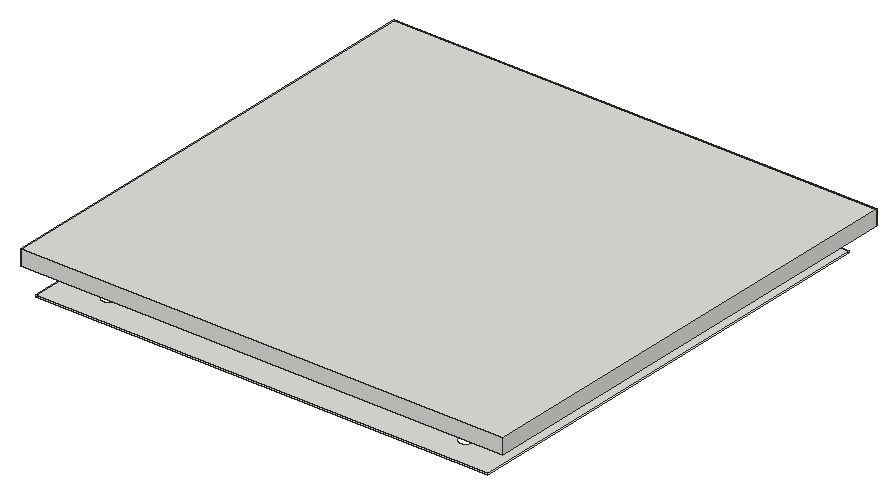
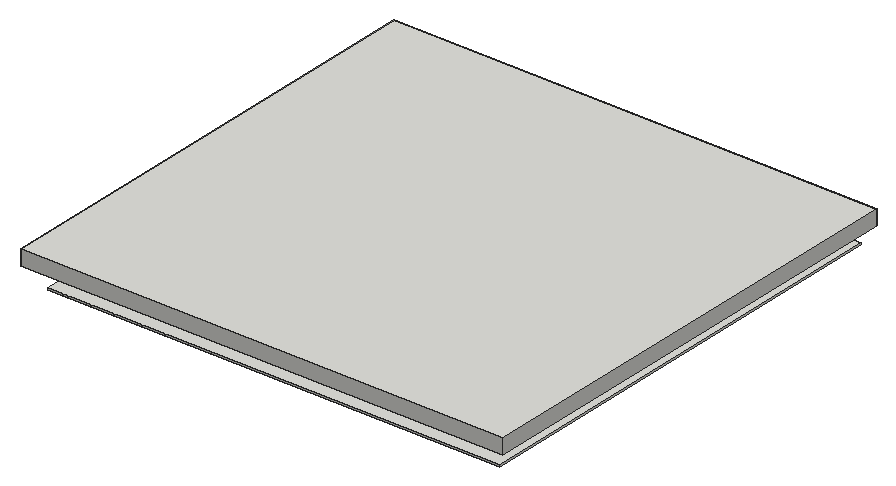
# SketchUp Ruby script. Lengths in inches.
U = 1.inch
M = Sketchup.active_model
def pt(a) = Geom::Point3d.new(a.map { |v| v * U })
def face(e, loops, mat)
  f = e.add_face(loops[0].map { |a| pt(a) })
  loops[1..].each { |l| e.add_face(l.map { |a| pt(a) }).erase! }
  f.material = f.back_material = mat if mat
  f
end
# faces: each face lists its corners as indices into pts; further lists are holes
def faces(e, pts, list, mat = nil) = list.each { |f| face(e, (f[0].is_a?(Array) ? f : [f]).map { |l| l.map { |i| pts[i] } }, mat) }
# xy, xz, yz: faces in a plane at the given z, y or x. An outline is a flat list of corners, or four numbers for a rectangle; further outlines are holes
def ring(l) = l.size == 4 ? [[l[0], l[1]], [l[2], l[1]], [l[2], l[3]], [l[0], l[3]]] : l.each_slice(2).to_a
def flat(e, list, mat, &to3) = list.each { |f| face(e, (f[0].is_a?(Array) ? f : [f]).map { |l| ring(l).map { |u, v| to3.(u, v) } }, mat) }
def xy(e, z, list, mat = nil) = flat(e, list, mat) { |x, y| [x, y, z] }
def xz(e, y, list, mat = nil) = flat(e, list, mat) { |x, z| [x, y, z] }
def yz(e, x, list, mat = nil) = flat(e, list, mat) { |y, z| [x, y, z] }
def lines(e, pts, list) = list.each { |a, b| e.add_line(pt(pts[a]), pt(pts[b])) }
# prism: a flat outline (further loops are holes) pulled along v
def prism(e, loops, v, mat = nil)
  f = face(e, loops, mat); d = Geom::Vector3d.new(v.map { |x| x * U })
  f.pushpull(f.normal.samedirection?(d) ? d.length : -d.length)
end
def box(e, o, s, mat = nil) = prism(e, [[o, [o[0] + s[0], o[1], o[2]], [o[0] + s[0], o[1] + s[1], o[2]], [o[0], o[1] + s[1], o[2]]]], [0, 0, s[2]], mat)
def at(x, y, z, deg = 0) = Geom::Transformation.translation(pt([x, y, z])) * Geom::Transformation.rotation(ORIGIN, Z_AXIS, deg.degrees)
def axes(o, x, y, z) = Geom::Transformation.new([*x, 0, *y, 0, *z, 0, *pt(o).to_a, 1])
def part(name) = M.definitions.add(name)
# library, detail: a bought-in or finely detailed component or shape, given as its bounding box
def library(name, o, s) = part(name).tap { |d| box(d.entities, o, s) }
def detail(e, o, s) = box(e.add_group.entities, o, s)
def put(e, d, t, mat = nil) = e.add_instance(d, t).tap { |i| i.material = mat if mat }
def group(e, t, mat = nil) = e.add_group.tap { |g| g.transformation = t; g.material = mat if mat }.entities
root = M.entities
xy(root,114,[[[4,0,124,120],[28,20,100,96],[112.03,72.63,112.26,72.64,112.48,72.68,112.71,72.74,112.92,72.83,113.125,72.9375,113.31,73.0625,113.49,73.21,113.65,73.375,113.8,73.56,113.92,73.75,114.02,73.96,114.1,74.17,114.16,74.4,114.19,74.625,114.2,74.86,114.18,75.08,114.15,75.3125,114.08,75.53,114,75.75,113.89,75.95,113.76,76.14,113.62,76.32,113.45,76.48,113.27,76.625,113.08,76.75,112.87,76.85,112.65,76.93,112.43,76.99,112.2,77.02,111.97,77.03,111.74,77.01,111.52,76.97,111.29,76.91,111.08,76.83,110.875,76.72,110.69,76.59,110.51,76.44,110.35,76.28,110.2,76.1,110.08,75.9,109.98,75.7,109.9,75.48,109.84,75.26,109.81,75.03,109.8,74.8,109.82,74.57,109.85,74.34,109.92,74.12,110,73.91,110.11,73.7,110.24,73.51,110.38,73.34,110.55,73.18,110.73,73.03,110.92,72.91,111.13,72.81,111.35,72.73,111.57,72.67,111.8,72.64],[112.03,106.04,112.26,106.06,112.48,106.1,112.71,106.16,112.92,106.24,113.125,106.35,113.31,106.48,113.49,106.625,113.65,106.79,113.8,106.97,113.92,107.17,114.02,107.37,114.1,107.59,114.16,107.8125,114.19,108.04,114.2,108.27,114.18,108.5,114.15,108.73,114.08,108.95,114,109.16,113.89,109.37,113.76,109.56,113.62,109.73,113.45,109.9,113.27,110.04,113.08,110.16,112.87,110.26,112.65,110.34,112.43,110.4,112.2,110.43,111.97,110.44,111.74,110.43,111.52,110.39,111.29,110.33,111.08,110.24,110.875,110.13,110.69,110.01,110.51,109.86,110.35,109.69,110.2,109.51,110.08,109.32,109.98,109.11,109.9,108.9,109.84,108.67,109.81,108.45,109.8,108.22,109.82,107.99,109.85,107.76,109.92,107.54,110,107.32,110.11,107.12,110.24,106.93,110.38,106.75,110.55,106.59,110.73,106.45,110.92,106.32,111.13,106.22,111.35,106.14,111.57,106.08,111.8,106.05],[112.03,39.21,112.26,39.23,112.48,39.27,112.71,39.33,112.92,39.42,113.125,39.52,113.31,39.65,113.49,39.8,113.65,39.96,113.8,40.14,113.92,40.34,114.02,40.54,114.1,40.76,114.16,40.98,114.19,41.21,114.2,41.44,114.18,41.67,114.15,41.9,114.08,42.12,114,42.33,113.89,42.54,113.76,42.73,113.62,42.91,113.45,43.07,113.27,43.21,113.08,43.33,112.87,43.43,112.65,43.51,112.43,43.57,112.2,43.6,111.97,43.61,111.74,43.6,111.52,43.56,111.29,43.5,111.08,43.41,110.875,43.31,110.69,43.18,110.51,43.03,110.35,42.87,110.2,42.69,110.08,42.49,109.98,42.28,109.9,42.07,109.84,41.85,109.81,41.62,109.8,41.39,109.82,41.16,109.85,40.93,109.92,40.71,110,40.49,110.11,40.29,110.24,40.1,110.38,39.92,110.55,39.76,110.73,39.62,110.92,39.5,111.13,39.39,111.35,39.3125,111.57,39.26,111.8,39.22],[112.03,5.8,112.26,5.82,112.48,5.85,112.71,5.92,112.92,6,113.125,6.11,113.31,6.24,113.49,6.38,113.65,6.55,113.8,6.73,113.92,6.92,114.02,7.13,114.1,7.35,114.16,7.57,114.19,7.8,114.2,8.03,114.18,8.26,114.15,8.48,114.08,8.71,114,8.92,113.89,9.125,113.76,9.31,113.62,9.49,113.45,9.65,113.27,9.8,113.08,9.92,112.87,10.02,112.65,10.1,112.43,10.16,112.2,10.19,111.97,10.2,111.74,10.18,111.52,10.15,111.29,10.08,111.08,10,110.875,9.89,110.69,9.76,110.51,9.62,110.35,9.45,110.2,9.27,110.08,9.08,109.98,8.87,109.9,8.65,109.84,8.43,109.81,8.2,109.8,7.97,109.82,7.74,109.85,7.52,109.92,7.29,110,7.08,110.11,6.875,110.24,6.69,110.38,6.51,110.55,6.35,110.73,6.2,110.92,6.08,111.13,5.98,111.35,5.9,111.57,5.84,111.8,5.81],[16.58,6.375,16.81,6.375,17.03,6.4,17.26,6.44,17.48,6.51,17.6875,6.6,17.89,6.72,18.07,6.85,18.25,7,18.4,7.17,18.54,7.36,18.65,7.56,18.75,7.77,18.82,7.98,18.87,8.21,18.89,8.4375,18.89,8.67,18.87,8.89,18.83,9.12,18.76,9.34,18.66,9.55,18.55,9.75,18.42,9.93,18.26,10.11,18.09,10.26,17.91,10.4,17.71,10.51,17.5,10.61,17.28,10.68,17.06,10.73,16.83,10.75,16.6,10.75,16.375,10.73,16.15,10.69,15.93,10.62,15.72,10.52,15.52,10.41,15.33,10.28,15.16,10.125,15.01,9.95,14.87,9.77,14.76,9.57,14.66,9.36,14.59,9.14,14.54,8.92,14.52,8.69,14.51,8.46,14.54,8.23,14.58,8.01,14.65,7.79,14.74,7.58,14.86,7.38,14.99,7.19,15.14,7.02,15.31,6.87,15.5,6.73,15.7,6.62,15.91,6.52,16.125,6.45,16.35,6.4],[16.58,39.72,16.81,39.72,17.03,39.74,17.26,39.79,17.48,39.86,17.6875,39.95,17.89,40.06,18.07,40.2,18.25,40.35,18.4,40.52,18.54,40.71,18.65,40.9,18.75,41.11,18.82,41.33,18.87,41.56,18.89,41.78,18.89,42.01,18.87,42.24,18.83,42.47,18.76,42.68,18.66,42.89,18.55,43.09,18.42,43.28,18.26,43.45,18.09,43.61,17.91,43.74,17.71,43.86,17.5,43.95,17.28,44.03,17.06,44.07,16.83,44.1,16.6,44.1,16.375,44.08,16.15,44.03,15.93,43.96,15.72,43.87,15.52,43.76,15.33,43.625,15.16,43.47,15.01,43.3,14.87,43.12,14.76,42.92,14.66,42.71,14.59,42.49,14.54,42.27,14.52,42.04,14.51,41.81,14.54,41.58,14.58,41.36,14.65,41.14,14.74,40.93,14.86,40.73,14.99,40.54,15.14,40.37,15.31,40.21,15.5,40.08,15.7,39.96,15.91,39.87,16.125,39.8,16.35,39.75],[16.58,73.07,16.81,73.07,17.03,73.09,17.26,73.14,17.48,73.21,17.6875,73.3,17.89,73.41,18.07,73.55,18.25,73.7,18.4,73.87,18.54,74.05,18.65,74.25,18.75,74.46,18.82,74.68,18.87,74.9,18.89,75.13,18.89,75.36,18.87,75.59,18.83,75.8125,18.76,76.03,18.66,76.24,18.55,76.44,18.42,76.63,18.26,76.8,18.09,76.95,17.91,77.09,17.71,77.21,17.5,77.3,17.28,77.37,17.06,77.42,16.83,77.45,16.6,77.45,16.375,77.43,16.15,77.38,15.93,77.31,15.72,77.22,15.52,77.1,15.33,76.97,15.16,76.82,15.01,76.65,14.87,76.46,14.76,76.26,14.66,76.06,14.59,75.84,14.54,75.61,14.52,75.39,14.51,75.16,14.54,74.93,14.58,74.7,14.65,74.48,14.74,74.27,14.86,74.07,14.99,73.89,15.14,73.72,15.31,73.5625,15.5,73.43,15.7,73.31,15.91,73.22,16.125,73.14,16.35,73.09],[16.81,106.41,17.03,106.4375,17.26,106.48,17.48,106.55,17.6875,106.65,17.89,106.76,18.07,106.89,18.25,107.05,18.4,107.21,18.54,107.4,18.65,107.6,18.75,107.81,18.82,108.02,18.87,108.25,18.89,108.48,18.89,108.71,18.87,108.94,18.83,109.16,18.76,109.38,18.66,109.59,18.55,109.79,18.42,109.97,18.26,110.15,18.09,110.3,17.91,110.4375,17.71,110.55,17.5,110.65,17.28,110.72,17.06,110.77,16.83,110.79,16.6,110.8,16.375,110.77,16.15,110.73,15.93,110.66,15.72,110.5625,15.52,110.45,15.33,110.32,15.16,110.16,15.01,109.99,14.87,109.81,14.76,109.61,14.66,109.4,14.59,109.18,14.54,108.96,14.52,108.73,14.51,108.5,14.54,108.27,14.58,108.05,14.65,107.83,14.74,107.62,14.86,107.42,14.99,107.23,15.14,107.0625,15.31,106.91,15.5,106.77,15.7,106.66,15.91,106.5625,16.125,106.49,16.35,106.44,16.58,106.42]]])
xy(root,114.34,[[16.59,73.27,16.38,73.29,16.18,73.34,15.98,73.4,15.79,73.49,15.61,73.59,15.44,73.72,15.29,73.86,15.15,74.01,15.03,74.18,14.92,74.36,14.84,74.55,14.78,74.75,14.73,74.96,14.71,75.17,14.72,75.375,14.74,75.58,14.78,75.78,14.85,75.98,14.93,76.17,15.04,76.35,15.16,76.52,15.3,76.68,15.46,76.8125,15.63,76.9375,15.81,77.04,16,77.12,16.2,77.1875,16.4,77.23,16.61,77.25,16.82,77.25,17.03,77.22,17.23,77.18,17.43,77.11,17.62,77.03,17.8,76.92,17.97,76.8,18.12,76.66,18.26,76.5,18.38,76.33,18.49,76.15,18.57,75.96,18.63,75.76,18.67,75.56,18.7,75.35,18.69,75.14,18.67,74.93,18.625,74.73,18.5625,74.53,18.47,74.34,18.37,74.16,18.25,73.99,18.11,73.84,17.95,73.7,17.78,73.58,17.6,73.48,17.41,73.39,17.21,73.33,17,73.29,16.8,73.27],[16.8,106.61,16.59,106.62,16.38,106.64,16.18,106.68,15.98,106.75,15.79,106.83,15.61,106.94,15.44,107.0625,15.29,107.2,15.15,107.36,15.03,107.53,14.92,107.71,14.84,107.9,14.78,108.1,14.73,108.3,14.71,108.51,14.72,108.72,14.74,108.93,14.78,109.13,14.85,109.33,14.93,109.52,15.04,109.7,15.16,109.87,15.3,110.02,15.46,110.16,15.63,110.28,15.81,110.39,16,110.47,16.2,110.53,16.4,110.57,16.61,110.6,16.82,110.59,17.03,110.57,17.23,110.53,17.43,110.46,17.62,110.375,17.8,110.27,17.97,110.15,18.12,110.01,18.26,109.85,18.38,109.68,18.49,109.5,18.57,109.31,18.63,109.11,18.67,108.9,18.7,108.7,18.69,108.49,18.67,108.28,18.625,108.08,18.5625,107.88,18.47,107.69,18.37,107.51,18.25,107.34,18.11,107.1875,17.95,107.05,17.78,106.93,17.6,106.82,17.41,106.74,17.21,106.68,17,106.63]])
xy(root,114.47,[[[4,0,124,120],[25.06,17.06,102.94,98.94],[112.02,106.24,111.82,106.25,111.61,106.28,111.41,106.33,111.21,106.41,111.02,106.5,110.84,106.61,110.68,106.74,110.53,106.89,110.4,107.05,110.28,107.22,110.18,107.41,110.11,107.6,110.05,107.8,110.01,108.01,110,108.22,110.01,108.43,110.04,108.63,110.09,108.84,110.16,109.03,110.26,109.22,110.37,109.4,110.5,109.5625,110.64,109.71,110.8,109.85,110.98,109.96,111.16,110.06,111.36,110.14,111.56,110.19,111.77,110.23,111.98,110.24,112.18,110.23,112.39,110.2,112.59,110.15,112.79,110.08,112.98,109.99,113.16,109.875,113.32,109.74,113.47,109.6,113.6,109.4375,113.72,109.26,113.82,109.08,113.89,108.88,113.95,108.68,113.99,108.48,114,108.27,113.99,108.06,113.96,107.85,113.91,107.65,113.84,107.45,113.74,107.26,113.63,107.09,113.5,106.92,113.36,106.77,113.2,106.64,113.02,106.52,112.84,106.43,112.64,106.35,112.44,106.29,112.23,106.26],[112.02,39.41,111.82,39.42,111.61,39.45,111.41,39.5,111.21,39.58,111.02,39.67,110.84,39.78,110.68,39.91,110.53,40.06,110.4,40.22,110.28,40.39,110.18,40.58,110.11,40.77,110.05,40.97,110.01,41.18,110,41.39,110.01,41.6,110.04,41.81,110.09,42.01,110.16,42.21,110.26,42.39,110.37,42.57,110.5,42.73,110.64,42.88,110.8,43.02,110.98,43.13,111.16,43.23,111.36,43.31,111.56,43.37,111.77,43.4,111.98,43.41,112.18,43.41,112.39,43.375,112.59,43.32,112.79,43.25,112.98,43.16,113.16,43.05,113.32,42.92,113.47,42.77,113.6,42.61,113.72,42.44,113.82,42.25,113.89,42.06,113.95,41.85,113.99,41.65,114,41.4375,113.99,41.23,113.96,41.02,113.91,40.82,113.84,40.625,113.74,40.44,113.63,40.26,113.5,40.09,113.36,39.94,113.2,39.8125,113.02,39.69,112.84,39.6,112.64,39.52,112.44,39.46,112.23,39.43],[112.02,6,111.82,6.01,111.61,6.04,111.41,6.09,111.21,6.16,111.02,6.26,110.84,6.37,110.68,6.5,110.53,6.64,110.4,6.8,110.28,6.98,110.18,7.16,110.11,7.36,110.05,7.56,110.01,7.77,110,7.98,110.01,8.18,110.04,8.39,110.09,8.59,110.16,8.79,110.26,8.98,110.37,9.16,110.5,9.32,110.64,9.47,110.8,9.6,110.98,9.72,111.16,9.82,111.36,9.89,111.56,9.95,111.77,9.99,111.98,10,112.18,9.99,112.39,9.96,112.59,9.91,112.79,9.84,112.98,9.74,113.16,9.63,113.32,9.5,113.47,9.36,113.6,9.2,113.72,9.02,113.82,8.84,113.89,8.64,113.95,8.44,113.99,8.23,114,8.02,113.99,7.82,113.96,7.61,113.91,7.41,113.84,7.21,113.74,7.02,113.63,6.84,113.5,6.68,113.36,6.53,113.2,6.4,113.02,6.28,112.84,6.18,112.64,6.11,112.44,6.05,112.23,6.01],[112.02,72.83,111.82,72.84,111.61,72.87,111.41,72.92,111.21,72.99,111.02,73.08,110.84,73.2,110.68,73.33,110.53,73.47,110.4,73.63,110.28,73.81,110.18,73.99,110.11,74.1875,110.05,74.39,110.01,74.59,110,74.8,110.01,75.01,110.04,75.22,110.09,75.42,110.16,75.62,110.26,75.81,110.37,75.98,110.5,76.15,110.64,76.3,110.8,76.43,110.98,76.55,111.16,76.65,111.36,76.72,111.56,76.78,111.77,76.8125,111.98,76.83,112.18,76.82,112.39,76.79,112.59,76.74,112.79,76.67,112.98,76.57,113.16,76.46,113.32,76.33,113.47,76.18,113.6,76.02,113.72,75.85,113.82,75.66,113.89,75.47,113.95,75.27,113.99,75.0625,114,74.85,113.99,74.64,113.96,74.4375,113.91,74.23,113.84,74.04,113.74,73.85,113.63,73.67,113.5,73.51,113.36,73.36,113.2,73.22,113.02,73.11,112.84,73.01,112.64,72.93,112.44,72.88,112.23,72.84],[16.59,39.92,16.38,39.94,16.18,39.99,15.98,40.05,15.79,40.14,15.61,40.25,15.44,40.37,15.29,40.51,15.15,40.67,15.03,40.84,14.92,41.02,14.84,41.21,14.78,41.41,14.73,41.61,14.71,41.82,14.72,42.03,14.74,42.23,14.78,42.4375,14.85,42.64,14.93,42.83,15.04,43.01,15.16,43.17,15.3,43.33,15.46,43.47,15.63,43.59,15.81,43.69,16,43.78,16.2,43.84,16.4,43.88,16.61,43.9,16.82,43.9,17.03,43.88,17.23,43.83,17.43,43.77,17.62,43.68,17.8,43.58,17.97,43.45,18.12,43.3125,18.26,43.16,18.38,42.99,18.49,42.81,18.57,42.61,18.63,42.42,18.67,42.21,18.7,42,18.69,41.79,18.67,41.59,18.625,41.38,18.5625,41.1875,18.47,41,18.37,40.82,18.25,40.65,18.11,40.49,17.95,40.35,17.78,40.23,17.6,40.13,17.41,40.05,17.21,39.98,17,39.94,16.8,39.92],[16.59,73.27,16.38,73.29,16.18,73.34,15.98,73.4,15.79,73.49,15.61,73.59,15.44,73.72,15.29,73.86,15.15,74.01,15.03,74.18,14.92,74.36,14.84,74.55,14.78,74.75,14.73,74.96,14.71,75.17,14.72,75.375,14.74,75.58,14.78,75.78,14.85,75.98,14.93,76.17,15.04,76.35,15.16,76.52,15.3,76.68,15.46,76.8125,15.63,76.9375,15.81,77.04,16,77.12,16.2,77.1875,16.4,77.23,16.61,77.25,16.82,77.25,17.03,77.22,17.23,77.18,17.43,77.11,17.62,77.03,17.8,76.92,17.97,76.8,18.12,76.66,18.26,76.5,18.38,76.33,18.49,76.15,18.57,75.96,18.63,75.76,18.67,75.56,18.7,75.35,18.69,75.14,18.67,74.93,18.625,74.73,18.5625,74.53,18.47,74.34,18.37,74.16,18.25,73.99,18.11,73.84,17.95,73.7,17.78,73.58,17.6,73.48,17.41,73.39,17.21,73.33,17,73.29,16.8,73.27],[16.59,6.57,16.38,6.6,16.18,6.64,15.98,6.71,15.79,6.79,15.61,6.9,15.44,7.02,15.29,7.16,15.15,7.32,15.03,7.49,14.92,7.67,14.84,7.86,14.78,8.06,14.73,8.26,14.71,8.47,14.72,8.68,14.74,8.89,14.78,9.09,14.85,9.29,14.93,9.48,15.04,9.66,15.16,9.83,15.3,9.98,15.46,10.12,15.63,10.24,15.81,10.34,16,10.43,16.2,10.49,16.4,10.53,16.61,10.55,16.82,10.55,17.03,10.53,17.23,10.49,17.43,10.42,17.62,10.33,17.8,10.23,17.97,10.11,18.12,9.96,18.26,9.81,18.38,9.64,18.49,9.46,18.57,9.27,18.63,9.07,18.67,8.86,18.7,8.66,18.69,8.45,18.67,8.24,18.625,8.04,18.5625,7.84,18.47,7.65,18.37,7.47,18.25,7.3,18.11,7.15,17.95,7.01,17.78,6.89,17.6,6.78,17.41,6.7,17.21,6.64,17,6.59,16.8,6.57],[16.8,106.61,16.59,106.62,16.38,106.64,16.18,106.68,15.98,106.75,15.79,106.83,15.61,106.94,15.44,107.0625,15.29,107.2,15.15,107.36,15.03,107.53,14.92,107.71,14.84,107.9,14.78,108.1,14.73,108.3,14.71,108.51,14.72,108.72,14.74,108.93,14.78,109.13,14.85,109.33,14.93,109.52,15.04,109.7,15.16,109.87,15.3,110.02,15.46,110.16,15.63,110.28,15.81,110.39,16,110.47,16.2,110.53,16.4,110.57,16.61,110.6,16.82,110.59,17.03,110.57,17.23,110.53,17.43,110.46,17.62,110.375,17.8,110.27,17.97,110.15,18.12,110.01,18.26,109.85,18.38,109.68,18.49,109.5,18.57,109.31,18.63,109.11,18.67,108.9,18.7,108.7,18.69,108.49,18.67,108.28,18.625,108.08,18.5625,107.88,18.47,107.69,18.37,107.51,18.25,107.34,18.11,107.1875,17.95,107.05,17.78,106.93,17.6,106.82,17.41,106.74,17.21,106.68,17,106.63]],[[25.53,17.53,102.47,98.47],[27.53,19.53,100.47,96.47]],[16.8,106.61,17,106.63,17.21,106.68,17.41,106.74,17.6,106.82,17.78,106.93,17.95,107.05,18.11,107.1875,18.25,107.34,18.37,107.51,18.47,107.69,18.5625,107.88,18.625,108.08,18.67,108.28,18.69,108.49,18.7,108.7,18.67,108.9,18.63,109.11,18.57,109.31,18.49,109.5,18.38,109.68,18.26,109.85,18.12,110.01,17.97,110.15,17.8,110.27,17.62,110.375,17.43,110.46,17.23,110.53,17.03,110.57,16.82,110.59,16.61,110.6,16.4,110.57,16.2,110.53,16,110.47,15.81,110.39,15.63,110.28,15.46,110.16,15.3,110.02,15.16,109.87,15.04,109.7,14.93,109.52,14.85,109.33,14.78,109.13,14.74,108.93,14.72,108.72,14.71,108.51,14.73,108.3,14.78,108.1,14.84,107.9,14.92,107.71,15.03,107.53,15.15,107.36,15.29,107.2,15.44,107.0625,15.61,106.94,15.79,106.83,15.98,106.75,16.18,106.68,16.38,106.64,16.59,106.62]])
xy(root,115.47,[[[27.53,19.53,100.47,96.47],[28,20,100,96]]])
xy(root,116.47,[[[25.06,17.06,102.94,98.94],[25.53,17.53,102.47,98.47]]])
xz(root,43.9,[[16.61,114.33,16.82,114.47]])
xz(root,73.27,[[16.59,114.34,16.8,114.47]])
xz(root,77.25,[[16.61,114.34,16.82,114.47]])
xz(root,96,[[28,114,100,115.47]])
xz(root,96.47,[[27.53,114.47,100.47,115.47]])
xz(root,98.47,[[25.53,114.47,102.47,116.47]])
xz(root,98.94,[[25.06,114.47,102.94,116.47]])
xz(root,120,[[4,114,124,114.47]])
yz(root,4,[[0,114,120,114.47]])
yz(root,25.06,[[17.06,114.47,98.94,116.47]])
yz(root,25.53,[[17.53,114.47,98.47,116.47]])
yz(root,27.53,[[19.53,114.47,96.47,115.47]])
yz(root,28,[[20,114,96,115.47]])
yz(root,100,[[20,114,96,115.47]])
yz(root,100.47,[[19.53,114.47,96.47,115.47]])
yz(root,102.47,[[17.53,114.47,98.47,116.47]])
yz(root,102.94,[[17.06,114.47,98.94,116.47]])
p = [[110.4,73.63,113.9],[110.28,73.81,113.9],[110.28,73.81,114.32],[110.4,73.63,114.32],[110.18,73.99,113.9],[110.18,73.99,114.32],
  [110.11,74.1875,113.9],[110.11,74.1875,114.32],[110.05,74.39,113.9],[110.05,74.39,114.32],[110.01,74.59,113.9],[110.01,74.59,114.32],
  [110,74.8,113.9],[110,74.8,114.32],[110.01,75.01,113.9],[110.01,75.01,114.32],[110.04,75.22,113.9],[110.04,75.22,114.32],
  [110.09,75.42,113.9],[110.09,75.42,114.32],[110.16,75.62,113.9],[110.16,75.62,114.32],[110.26,75.81,113.9],[110.26,75.81,114.32],
  [110.37,75.98,113.9],[110.37,75.98,114.32],[110.28,107.22,113.9],[110.18,107.41,113.9],[110.18,107.41,114.32],[110.28,107.22,114.32],
  [110.11,107.6,113.9],[110.11,107.6,114.32],[110.05,107.8,113.9],[110.05,107.8,114.32],[110.01,108.01,113.9],[110.01,108.01,114.32],
  [110,108.22,113.9],[110,108.22,114.32],[110.01,108.43,113.9],[110.01,108.43,114.32],[110.04,108.63,113.9],[110.04,108.63,114.32],
  [110.09,108.84,113.9],[110.09,108.84,114.32],[110.16,109.03,113.9],[110.16,109.03,114.32],[110.26,109.22,113.9],[110.26,109.22,114.32],
  [110.37,109.4,113.9],[110.37,109.4,114.32],[15.81,43.69,114.47],[15.81,43.69,114.33],[16,43.78,114.33],[16,43.78,114.47],
  [17.43,43.77,114.47],[17.43,43.77,114.33],[17.62,43.68,114.33],[17.62,43.68,114.47],[16.2,43.84,114.33],[16.2,43.84,114.47],
  [16.4,43.88,114.33],[16.4,43.88,114.47],[17.03,43.88,114.47],[17.03,43.88,114.33],[17.23,43.83,114.33],[17.23,43.83,114.47],
  [16.61,43.9,114.33],[16.61,43.9,114.47],[16.82,43.9,114.47],[16.82,43.9,114.33],[16.18,73.34,114.47],[16.18,73.34,114.34],
  [15.98,73.4,114.34],[15.98,73.4,114.47],[16.38,73.29,114.47],[16.38,73.29,114.34],[16.59,73.27,114.47],[16.59,73.27,114.34],
  [17,73.29,114.47],[17,73.29,114.34],[16.8,73.27,114.34],[16.8,73.27,114.47],[17.21,73.33,114.47],[17.21,73.33,114.34],
  [17.41,73.39,114.47],[17.41,73.39,114.34],[15.79,73.49,114.34],[15.79,73.49,114.47],[17.6,73.48,114.47],[17.6,73.48,114.34],
  [15.61,73.59,114.34],[15.61,73.59,114.47],[17.78,73.58,114.47],[17.78,73.58,114.34],[15.44,73.72,114.34],[15.44,73.72,114.47],
  [17.95,73.7,114.47],[17.95,73.7,114.34],[15.29,73.86,114.34],[15.29,73.86,114.47],[18.11,73.84,114.47],[18.11,73.84,114.34],
  [18.25,73.99,114.47],[18.25,73.99,114.34],[110.28,73.81,114.47],[110.18,73.99,114.47],[15.15,74.01,114.34],[15.15,74.01,114.47],
  [15.03,74.18,114.34],[15.03,74.18,114.47],[18.37,74.16,114.47],[18.37,74.16,114.34],[110.11,74.1875,114.47],[14.92,74.36,114.34],
  [14.92,74.36,114.47],[18.47,74.34,114.47],[18.47,74.34,114.34],[110.05,74.39,114.47],[18.5625,74.53,114.47],[18.5625,74.53,114.34],
  [14.84,74.55,114.34],[14.84,74.55,114.47],[110.01,74.59,114.47],[18.625,74.73,114.47],[18.625,74.73,114.34],[14.78,74.75,114.34],
  [14.78,74.75,114.47],[110,74.8,114.47],[18.67,74.93,114.47],[18.67,74.93,114.34],[14.73,74.96,114.34],[14.73,74.96,114.47],
  [110.01,75.01,114.47],[18.69,75.14,114.47],[18.69,75.14,114.34],[14.71,75.17,114.34],[14.71,75.17,114.47],[110.04,75.22,114.47],
  [18.7,75.35,114.47],[18.7,75.35,114.34],[14.72,75.375,114.34],[14.72,75.375,114.47],[110.09,75.42,114.47],[14.74,75.58,114.34],
  [14.74,75.58,114.47],[18.67,75.56,114.47],[18.67,75.56,114.34],[110.16,75.62,114.47],[14.78,75.78,114.34],[14.78,75.78,114.47],
  [18.63,75.76,114.47],[18.63,75.76,114.34],[110.26,75.81,114.47],[14.85,75.98,114.34],[14.85,75.98,114.47],[18.57,75.96,114.47],
  [18.57,75.96,114.34],[110.37,75.98,114.47],[14.93,76.17,114.34],[14.93,76.17,114.47],[18.49,76.15,114.47],[18.49,76.15,114.34],
  [15.04,76.35,114.34],[15.04,76.35,114.47],[18.38,76.33,114.47],[18.38,76.33,114.34],[18.26,76.5,114.47],[18.26,76.5,114.34],
  [15.16,76.52,114.34],[15.16,76.52,114.47],[15.3,76.68,114.34],[15.3,76.68,114.47],[18.12,76.66,114.47],[18.12,76.66,114.34],
  [15.46,76.8125,114.34],[15.46,76.8125,114.47],[17.97,76.8,114.47],[17.97,76.8,114.34],[15.63,76.9375,114.34],[15.63,76.9375,114.47],
  [17.8,76.92,114.47],[17.8,76.92,114.34],[15.81,77.04,114.34],[15.81,77.04,114.47],[17.62,77.03,114.47],[17.62,77.03,114.34],
  [16,77.12,114.34],[16,77.12,114.47],[17.43,77.11,114.47],[17.43,77.11,114.34],[16.2,77.1875,114.34],[16.2,77.1875,114.47],
  [17.23,77.18,114.47],[17.23,77.18,114.34],[16.4,77.23,114.34],[16.4,77.23,114.47],[16.61,77.25,114.34],[16.61,77.25,114.47],
  [16.82,77.25,114.47],[16.82,77.25,114.34],[17.03,77.22,114.34],[17.03,77.22,114.47],[16.38,106.64,114.47],[16.38,106.64,114.34],
  [16.18,106.68,114.34],[16.18,106.68,114.47],[16.59,106.62,114.47],[16.59,106.62,114.34],[16.8,106.61,114.47],[16.8,106.61,114.34],
  [17,106.63,114.47],[17,106.63,114.34],[17.21,106.68,114.47],[17.21,106.68,114.34],[15.98,106.75,114.47],[15.98,106.75,114.34],
  [15.79,106.83,114.34],[15.79,106.83,114.47],[17.41,106.74,114.47],[17.41,106.74,114.34],[17.6,106.82,114.47],[17.6,106.82,114.34],
  [15.61,106.94,114.34],[15.61,106.94,114.47],[17.78,106.93,114.47],[17.78,106.93,114.34],[15.44,107.0625,114.34],[15.44,107.0625,114.47],
  [17.95,107.05,114.47],[17.95,107.05,114.34],[18.11,107.1875,114.47],[18.11,107.1875,114.34],[15.29,107.2,114.34],[15.29,107.2,114.47],
  [15.15,107.36,114.34],[15.15,107.36,114.47],[18.25,107.34,114.47],[18.25,107.34,114.34],[110.28,107.22,114.47],[110.18,107.41,114.47],
  [18.37,107.51,114.47],[18.37,107.51,114.34],[15.03,107.53,114.34],[15.03,107.53,114.47],[110.11,107.6,114.47],[14.92,107.71,114.34],
  [14.92,107.71,114.47],[18.47,107.69,114.47],[18.47,107.69,114.34],[110.05,107.8,114.47],[14.84,107.9,114.34],[14.84,107.9,114.47],
  [18.5625,107.88,114.47],[18.5625,107.88,114.34],[110.01,108.01,114.47],[14.78,108.1,114.34],[14.78,108.1,114.47],[18.625,108.08,114.47],
  [18.625,108.08,114.34],[110,108.22,114.47],[14.73,108.3,114.34],[14.73,108.3,114.47],[18.67,108.28,114.47],[18.67,108.28,114.34],
  [110.01,108.43,114.47],[14.71,108.51,114.34],[14.71,108.51,114.47],[18.69,108.49,114.47],[18.69,108.49,114.34],[110.04,108.63,114.47],
  [14.72,108.72,114.34],[14.72,108.72,114.47],[18.7,108.7,114.47],[18.7,108.7,114.34],[110.09,108.84,114.47],[14.74,108.93,114.34],
  [14.74,108.93,114.47],[18.67,108.9,114.47],[18.67,108.9,114.34],[110.16,109.03,114.47],[14.78,109.13,114.34],[14.78,109.13,114.47],
  [18.63,109.11,114.47],[18.63,109.11,114.34],[110.26,109.22,114.47],[14.85,109.33,114.34],[14.85,109.33,114.47],[18.57,109.31,114.47],
  [18.57,109.31,114.34],[110.37,109.4,114.47],[14.93,109.52,114.34],[14.93,109.52,114.47],[18.49,109.5,114.47],[18.49,109.5,114.34],
  [15.04,109.7,114.34],[15.04,109.7,114.47],[18.38,109.68,114.47],[18.38,109.68,114.34],[15.16,109.87,114.34],[15.16,109.87,114.47],
  [18.26,109.85,114.47],[18.26,109.85,114.34],[18.12,110.01,114.47],[18.12,110.01,114.34],[15.3,110.02,114.34],[15.3,110.02,114.47],
  [15.46,110.16,114.34],[15.46,110.16,114.47],[17.97,110.15,114.47],[17.97,110.15,114.34],[17.8,110.27,114.47],[17.8,110.27,114.34],
  [15.63,110.28,114.34],[15.63,110.28,114.47],[15.81,110.39,114.34],[15.81,110.39,114.47],[17.62,110.375,114.47],[17.62,110.375,114.34],
  [16,110.47,114.34],[16,110.47,114.47],[17.43,110.46,114.47],[17.43,110.46,114.34],[16.2,110.53,114.34],[16.2,110.53,114.47],
  [16.4,110.57,114.34],[16.4,110.57,114.47],[17.03,110.57,114.47],[17.03,110.57,114.34],[17.23,110.53,114.34],[17.23,110.53,114.47],
  [16.61,110.6,114.34],[16.61,110.6,114.47],[16.82,110.59,114.34],[16.82,110.59,114.47]]
faces(root,p,[[0,1,2,3],[1,4,5,2],[4,6,7,5],[6,8,9,7],[8,10,11,9],[10,12,13,11],[12,14,15,13],[14,16,17,15],
  [16,18,19,17],[18,20,21,19],[20,22,23,21],[22,24,25,23],[26,27,28,29],[27,30,31,28],[30,32,33,31],[32,34,35,33],
  [34,36,37,35],[36,38,39,37],[38,40,41,39],[40,42,43,41],[42,44,45,43],[44,46,47,45],[46,48,49,47],[50,51,52,53],
  [54,55,56,57],[53,52,58,59],[59,58,60,61],[62,63,64,65],[65,64,55,54],[61,60,66,67],[68,69,63,62],[70,71,72,73],
  [74,75,71,70],[76,77,75,74],[78,79,80,81],[82,83,79,78],[84,85,83,82],[73,72,86,87],[88,89,85,84],[87,86,90,91],
  [92,93,89,88],[91,90,94,95],[96,97,93,92],[95,94,98,99],[100,101,97,96],[102,103,101,100],[104,2,5,105],[99,98,106,107],
  [107,106,108,109],[110,111,103,102],[105,5,7,112],[109,108,113,114],[115,116,111,110],[112,7,9,117],[118,119,116,115],[114,113,120,121],
  [117,9,11,122],[123,124,119,118],[121,120,125,126],[122,11,13,127],[128,129,124,123],[126,125,130,131],[127,13,15,132],[133,134,129,128],
  [131,130,135,136],[132,15,17,137],[138,139,134,133],[136,135,140,141],[137,17,19,142],[141,140,143,144],[145,146,139,138],[142,19,21,147],
  [144,143,148,149],[150,151,146,145],[147,21,23,152],[149,148,153,154],[155,156,151,150],[152,23,25,157],[154,153,158,159],[160,161,156,155],
  [159,158,162,163],[164,165,161,160],[166,167,165,164],[163,162,168,169],[169,168,170,171],[172,173,167,166],[171,170,174,175],[176,177,173,172],
  [175,174,178,179],[180,181,177,176],[179,178,182,183],[184,185,181,180],[183,182,186,187],[188,189,185,184],[187,186,190,191],[192,193,189,188],
  [191,190,194,195],[195,194,196,197],[198,199,200,201],[201,200,193,192],[202,203,204,205],[206,207,203,202],[208,209,207,206],[210,211,209,208],
  [212,213,211,210],[214,215,216,217],[205,204,215,214],[218,219,213,212],[220,221,219,218],[217,216,222,223],[224,225,221,220],[223,222,226,227],
  [228,229,225,224],[230,231,229,228],[227,226,232,233],[233,232,234,235],[236,237,231,230],[238,29,28,239],[240,241,237,236],[235,234,242,243],
  [239,28,31,244],[243,242,245,246],[247,248,241,240],[244,31,33,249],[246,245,250,251],[252,253,248,247],[249,33,35,254],[251,250,255,256],
  [257,258,253,252],[254,35,37,259],[256,255,260,261],[262,263,258,257],[259,37,39,264],[261,260,265,266],[267,268,263,262],[264,39,41,269],
  [266,265,270,271],[272,273,268,267],[269,41,43,274],[271,270,275,276],[277,278,273,272],[274,43,45,279],[276,275,280,281],[282,283,278,277],
  [279,45,47,284],[281,280,285,286],[287,288,283,282],[284,47,49,289],[286,285,290,291],[292,293,288,287],[291,290,294,295],[296,297,293,292],
  [295,294,298,299],[300,301,297,296],[302,303,301,300],[299,298,304,305],[305,304,306,307],[308,309,303,302],[310,311,309,308],[307,306,312,313],
  [313,312,314,315],[316,317,311,310],[315,314,318,319],[320,321,317,316],[319,318,322,323],[323,322,324,325],[326,327,328,329],[329,328,321,320],
  [325,324,330,331],[331,330,332,333],[333,332,327,326]])
g1 = group(root,at(0,0,120))
box(g1,[0,0,0],[128,124,4])
g2 = group(root,at(25.06,17.06,116.47))
box(g2,[0,0,0],[77.89,81.89,0.47])
